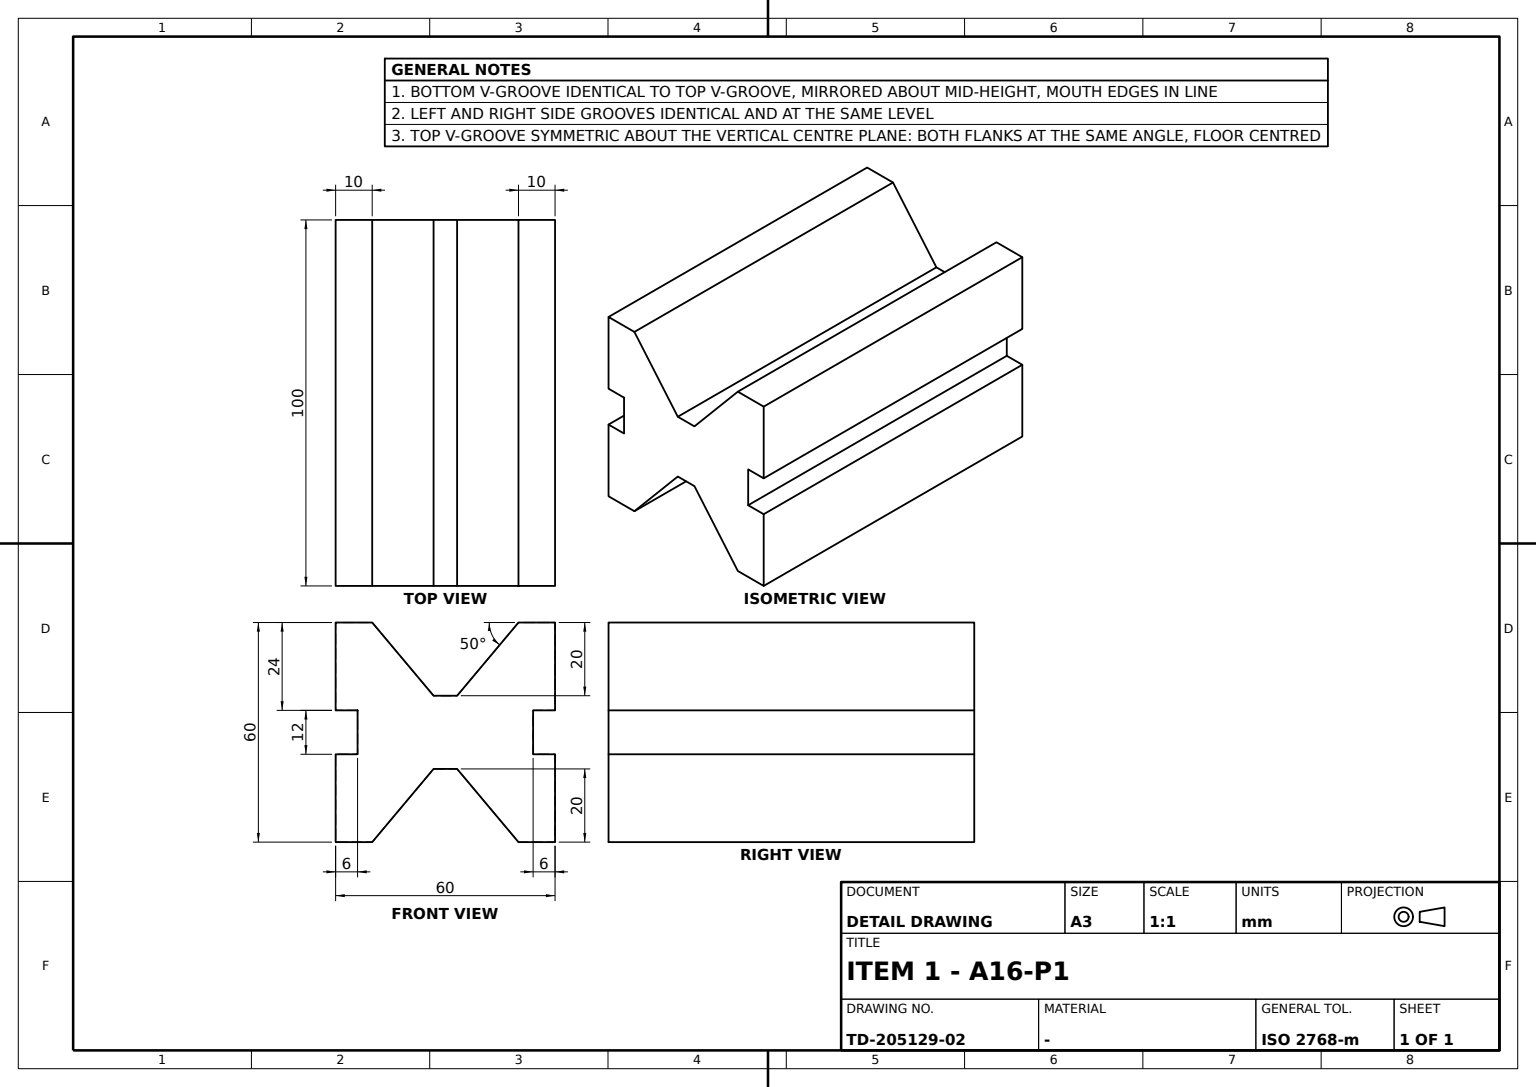
ISO-10303-21;
HEADER;
FILE_DESCRIPTION((''),'2;1');
FILE_NAME('','',(''),(''),'','','');
FILE_SCHEMA(('AUTOMOTIVE_DESIGN'));
ENDSEC;
DATA;
#1=APPLICATION_CONTEXT('');
#2=PRODUCT_CONTEXT('',#1,'mechanical');
#3=PRODUCT('','','',(#2));
#4=PRODUCT_DEFINITION_FORMATION('','',#3);
#5=PRODUCT_DEFINITION_CONTEXT('',#1,'design');
#6=PRODUCT_DEFINITION('','',#4,#5);
#7=PRODUCT_DEFINITION_SHAPE('','',#6);
#8=(LENGTH_UNIT()NAMED_UNIT(*)SI_UNIT(.MILLI.,.METRE.));
#9=(NAMED_UNIT(*)PLANE_ANGLE_UNIT()SI_UNIT($,.RADIAN.));
#10=(NAMED_UNIT(*)SI_UNIT($,.STERADIAN.)SOLID_ANGLE_UNIT());
#11=UNCERTAINTY_MEASURE_WITH_UNIT(LENGTH_MEASURE(0.005),#8,'distance_accuracy_value','');
#12=(GEOMETRIC_REPRESENTATION_CONTEXT(3)GLOBAL_UNCERTAINTY_ASSIGNED_CONTEXT((#11))GLOBAL_UNIT_ASSIGNED_CONTEXT((#8,#9,#10))REPRESENTATION_CONTEXT('',''));
#13=CARTESIAN_POINT('',(100.,30.,-6.));
#14=VERTEX_POINT('',#13);
#15=CARTESIAN_POINT('',(100.,24.,-6.));
#16=VERTEX_POINT('',#15);
#17=CARTESIAN_POINT('',(100.,0.,-6.));
#18=DIRECTION('',(0.,-1.,0.));
#19=VECTOR('',#18,1000.);
#20=LINE('',#17,#19);
#21=EDGE_CURVE('',#14,#16,#20,.T.);
#22=ORIENTED_EDGE('',*,*,#21,.F.);
#23=CARTESIAN_POINT('',(0.,30.,-6.));
#24=VERTEX_POINT('',#23);
#25=DIRECTION('',(1.,0.,0.));
#26=VECTOR('',#25,1000.);
#27=LINE('',#23,#26);
#28=EDGE_CURVE('',#24,#14,#27,.T.);
#29=ORIENTED_EDGE('',*,*,#28,.F.);
#30=CARTESIAN_POINT('',(0.,24.,-6.));
#31=VERTEX_POINT('',#30);
#32=CARTESIAN_POINT('',(0.,0.,-6.));
#33=LINE('',#32,#19);
#34=EDGE_CURVE('',#24,#31,#33,.T.);
#35=ORIENTED_EDGE('',*,*,#34,.T.);
#36=LINE('',#30,#26);
#37=EDGE_CURVE('',#31,#16,#36,.T.);
#38=ORIENTED_EDGE('',*,*,#37,.T.);
#39=EDGE_LOOP('',(#22,#29,#35,#38));
#40=FACE_BOUND('',#39,.T.);
#41=CARTESIAN_POINT('',(0.,-24.,-6.));
#42=DIRECTION('',(0.,0.,1.));
#43=AXIS2_PLACEMENT_3D('',#41,#42,#18);
#44=PLANE('',#43);
#45=ADVANCED_FACE('',(#40),#44,.T.);
#46=CARTESIAN_POINT('',(100.,-30.,-6.));
#47=VERTEX_POINT('',#46);
#48=CARTESIAN_POINT('',(100.,-30.,-30.));
#49=VERTEX_POINT('',#48);
#50=CARTESIAN_POINT('',(100.,-30.,0.));
#51=DIRECTION('',(0.,0.,-1.));
#52=VECTOR('',#51,1000.);
#53=LINE('',#50,#52);
#54=EDGE_CURVE('',#47,#49,#53,.T.);
#55=ORIENTED_EDGE('',*,*,#54,.F.);
#56=CARTESIAN_POINT('',(0.,-30.,-6.));
#57=VERTEX_POINT('',#56);
#58=LINE('',#56,#26);
#59=EDGE_CURVE('',#57,#47,#58,.T.);
#60=ORIENTED_EDGE('',*,*,#59,.F.);
#61=CARTESIAN_POINT('',(0.,-30.,-30.));
#62=VERTEX_POINT('',#61);
#63=CARTESIAN_POINT('',(0.,-30.,0.));
#64=LINE('',#63,#52);
#65=EDGE_CURVE('',#57,#62,#64,.T.);
#66=ORIENTED_EDGE('',*,*,#65,.T.);
#67=LINE('',#61,#26);
#68=EDGE_CURVE('',#62,#49,#67,.T.);
#69=ORIENTED_EDGE('',*,*,#68,.T.);
#70=EDGE_LOOP('',(#55,#60,#66,#69));
#71=FACE_BOUND('',#70,.T.);
#72=AXIS2_PLACEMENT_3D('',#56,#18,#51);
#73=PLANE('',#72);
#74=ADVANCED_FACE('',(#71),#73,.T.);
#75=CARTESIAN_POINT('',(0.,30.,30.));
#76=VERTEX_POINT('',#75);
#77=CARTESIAN_POINT('',(0.,30.,6.));
#78=VERTEX_POINT('',#77);
#79=CARTESIAN_POINT('',(0.,30.,-30.));
#80=LINE('',#79,#52);
#81=EDGE_CURVE('',#76,#78,#80,.T.);
#82=ORIENTED_EDGE('',*,*,#81,.F.);
#83=CARTESIAN_POINT('',(100.,30.,30.));
#84=VERTEX_POINT('',#83);
#85=LINE('',#75,#26);
#86=EDGE_CURVE('',#76,#84,#85,.T.);
#87=ORIENTED_EDGE('',*,*,#86,.T.);
#88=CARTESIAN_POINT('',(100.,30.,6.));
#89=VERTEX_POINT('',#88);
#90=CARTESIAN_POINT('',(100.,30.,-30.));
#91=LINE('',#90,#52);
#92=EDGE_CURVE('',#84,#89,#91,.T.);
#93=ORIENTED_EDGE('',*,*,#92,.T.);
#94=LINE('',#77,#26);
#95=EDGE_CURVE('',#78,#89,#94,.T.);
#96=ORIENTED_EDGE('',*,*,#95,.F.);
#97=EDGE_LOOP('',(#82,#87,#93,#96));
#98=FACE_BOUND('',#97,.T.);
#99=DIRECTION('',(0.,1.,0.));
#100=AXIS2_PLACEMENT_3D('',#79,#99,#42);
#101=PLANE('',#100);
#102=ADVANCED_FACE('',(#98),#101,.T.);
#103=VERTEX_POINT('',#41);
#104=CARTESIAN_POINT('',(100.,-24.,-6.));
#105=VERTEX_POINT('',#104);
#106=LINE('',#41,#26);
#107=EDGE_CURVE('',#103,#105,#106,.T.);
#108=ORIENTED_EDGE('',*,*,#107,.F.);
#109=EDGE_CURVE('',#103,#57,#33,.T.);
#110=ORIENTED_EDGE('',*,*,#109,.T.);
#111=ORIENTED_EDGE('',*,*,#59,.T.);
#112=EDGE_CURVE('',#105,#47,#20,.T.);
#113=ORIENTED_EDGE('',*,*,#112,.F.);
#114=EDGE_LOOP('',(#108,#110,#111,#113));
#115=FACE_BOUND('',#114,.T.);
#116=ADVANCED_FACE('',(#115),#44,.T.);
#117=CARTESIAN_POINT('',(0.,3.218007,10.));
#118=VERTEX_POINT('',#117);
#119=CARTESIAN_POINT('',(100.,3.218007,10.));
#120=VERTEX_POINT('',#119);
#121=LINE('',#117,#26);
#122=EDGE_CURVE('',#118,#120,#121,.T.);
#123=ORIENTED_EDGE('',*,*,#122,.F.);
#124=CARTESIAN_POINT('',(0.,-3.218007,10.));
#125=VERTEX_POINT('',#124);
#126=CARTESIAN_POINT('',(0.,0.,10.));
#127=VECTOR('',#99,1000.);
#128=LINE('',#126,#127);
#129=EDGE_CURVE('',#125,#118,#128,.T.);
#130=ORIENTED_EDGE('',*,*,#129,.F.);
#131=CARTESIAN_POINT('',(100.,-3.218007,10.));
#132=VERTEX_POINT('',#131);
#133=LINE('',#124,#26);
#134=EDGE_CURVE('',#125,#132,#133,.T.);
#135=ORIENTED_EDGE('',*,*,#134,.T.);
#136=CARTESIAN_POINT('',(100.,0.,10.));
#137=LINE('',#136,#127);
#138=EDGE_CURVE('',#132,#120,#137,.T.);
#139=ORIENTED_EDGE('',*,*,#138,.T.);
#140=EDGE_LOOP('',(#123,#130,#135,#139));
#141=FACE_BOUND('',#140,.T.);
#142=AXIS2_PLACEMENT_3D('',#124,#51,#99);
#143=PLANE('',#142);
#144=ADVANCED_FACE('',(#141),#143,.F.);
#145=ORIENTED_EDGE('',*,*,#122,.T.);
#146=CARTESIAN_POINT('',(100.,20.,30.));
#147=VERTEX_POINT('',#146);
#148=CARTESIAN_POINT('',(100.,-3.035635,2.5472));
#149=DIRECTION('',(0.,0.64278761,0.766044443));
#150=VECTOR('',#149,1000.);
#151=LINE('',#148,#150);
#152=EDGE_CURVE('',#120,#147,#151,.T.);
#153=ORIENTED_EDGE('',*,*,#152,.T.);
#154=CARTESIAN_POINT('',(0.,20.,30.));
#155=VERTEX_POINT('',#154);
#156=LINE('',#154,#26);
#157=EDGE_CURVE('',#155,#147,#156,.T.);
#158=ORIENTED_EDGE('',*,*,#157,.F.);
#159=CARTESIAN_POINT('',(0.,-3.035635,2.5472));
#160=LINE('',#159,#150);
#161=EDGE_CURVE('',#118,#155,#160,.T.);
#162=ORIENTED_EDGE('',*,*,#161,.F.);
#163=EDGE_LOOP('',(#145,#153,#158,#162));
#164=FACE_BOUND('',#163,.T.);
#165=DIRECTION('',(0.,0.766044443,-0.64278761));
#166=AXIS2_PLACEMENT_3D('',#117,#165,#149);
#167=PLANE('',#166);
#168=ADVANCED_FACE('',(#164),#167,.F.);
#169=CARTESIAN_POINT('',(0.,-30.,30.));
#170=VERTEX_POINT('',#169);
#171=CARTESIAN_POINT('',(100.,-30.,30.));
#172=VERTEX_POINT('',#171);
#173=LINE('',#169,#26);
#174=EDGE_CURVE('',#170,#172,#173,.T.);
#175=ORIENTED_EDGE('',*,*,#174,.T.);
#176=CARTESIAN_POINT('',(100.,-20.,30.));
#177=VERTEX_POINT('',#176);
#178=CARTESIAN_POINT('',(100.,0.,30.));
#179=LINE('',#178,#127);
#180=EDGE_CURVE('',#172,#177,#179,.T.);
#181=ORIENTED_EDGE('',*,*,#180,.T.);
#182=CARTESIAN_POINT('',(0.,-20.,30.));
#183=VERTEX_POINT('',#182);
#184=LINE('',#182,#26);
#185=EDGE_CURVE('',#183,#177,#184,.T.);
#186=ORIENTED_EDGE('',*,*,#185,.F.);
#187=CARTESIAN_POINT('',(0.,0.,30.));
#188=LINE('',#187,#127);
#189=EDGE_CURVE('',#170,#183,#188,.T.);
#190=ORIENTED_EDGE('',*,*,#189,.F.);
#191=EDGE_LOOP('',(#175,#181,#186,#190));
#192=FACE_BOUND('',#191,.T.);
#193=AXIS2_PLACEMENT_3D('',#154,#51,#99);
#194=PLANE('',#193);
#195=ADVANCED_FACE('',(#192),#194,.F.);
#196=CARTESIAN_POINT('',(100.,-24.,6.));
#197=VERTEX_POINT('',#196);
#198=CARTESIAN_POINT('',(100.,-30.,6.));
#199=VERTEX_POINT('',#198);
#200=CARTESIAN_POINT('',(100.,0.,6.));
#201=LINE('',#200,#19);
#202=EDGE_CURVE('',#197,#199,#201,.T.);
#203=ORIENTED_EDGE('',*,*,#202,.T.);
#204=CARTESIAN_POINT('',(0.,-30.,6.));
#205=VERTEX_POINT('',#204);
#206=LINE('',#204,#26);
#207=EDGE_CURVE('',#205,#199,#206,.T.);
#208=ORIENTED_EDGE('',*,*,#207,.F.);
#209=CARTESIAN_POINT('',(0.,-24.,6.));
#210=VERTEX_POINT('',#209);
#211=CARTESIAN_POINT('',(0.,0.,6.));
#212=LINE('',#211,#19);
#213=EDGE_CURVE('',#210,#205,#212,.T.);
#214=ORIENTED_EDGE('',*,*,#213,.F.);
#215=LINE('',#209,#26);
#216=EDGE_CURVE('',#210,#197,#215,.T.);
#217=ORIENTED_EDGE('',*,*,#216,.T.);
#218=EDGE_LOOP('',(#203,#208,#214,#217));
#219=FACE_BOUND('',#218,.T.);
#220=AXIS2_PLACEMENT_3D('',#77,#42,#18);
#221=PLANE('',#220);
#222=ADVANCED_FACE('',(#219),#221,.F.);
#223=ORIENTED_EDGE('',*,*,#68,.F.);
#224=CARTESIAN_POINT('',(0.,-20.,-30.));
#225=VERTEX_POINT('',#224);
#226=CARTESIAN_POINT('',(0.,0.,-30.));
#227=LINE('',#226,#127);
#228=EDGE_CURVE('',#62,#225,#227,.T.);
#229=ORIENTED_EDGE('',*,*,#228,.T.);
#230=CARTESIAN_POINT('',(100.,-20.,-30.));
#231=VERTEX_POINT('',#230);
#232=LINE('',#224,#26);
#233=EDGE_CURVE('',#225,#231,#232,.T.);
#234=ORIENTED_EDGE('',*,*,#233,.T.);
#235=CARTESIAN_POINT('',(100.,0.,-30.));
#236=LINE('',#235,#127);
#237=EDGE_CURVE('',#49,#231,#236,.T.);
#238=ORIENTED_EDGE('',*,*,#237,.F.);
#239=EDGE_LOOP('',(#223,#229,#234,#238));
#240=FACE_BOUND('',#239,.T.);
#241=AXIS2_PLACEMENT_3D('',#61,#51,#99);
#242=PLANE('',#241);
#243=ADVANCED_FACE('',(#240),#242,.T.);
#244=CARTESIAN_POINT('',(0.,20.,-30.));
#245=VERTEX_POINT('',#244);
#246=CARTESIAN_POINT('',(100.,20.,-30.));
#247=VERTEX_POINT('',#246);
#248=LINE('',#244,#26);
#249=EDGE_CURVE('',#245,#247,#248,.T.);
#250=ORIENTED_EDGE('',*,*,#249,.F.);
#251=VERTEX_POINT('',#79);
#252=EDGE_CURVE('',#245,#251,#227,.T.);
#253=ORIENTED_EDGE('',*,*,#252,.T.);
#254=VERTEX_POINT('',#90);
#255=LINE('',#79,#26);
#256=EDGE_CURVE('',#251,#254,#255,.T.);
#257=ORIENTED_EDGE('',*,*,#256,.T.);
#258=EDGE_CURVE('',#247,#254,#236,.T.);
#259=ORIENTED_EDGE('',*,*,#258,.F.);
#260=EDGE_LOOP('',(#250,#253,#257,#259));
#261=FACE_BOUND('',#260,.T.);
#262=ADVANCED_FACE('',(#261),#242,.T.);
#263=VECTOR('',#42,1000.);
#264=LINE('',#56,#263);
#265=EDGE_CURVE('',#205,#170,#264,.T.);
#266=ORIENTED_EDGE('',*,*,#265,.F.);
#267=ORIENTED_EDGE('',*,*,#207,.T.);
#268=LINE('',#46,#263);
#269=EDGE_CURVE('',#199,#172,#268,.T.);
#270=ORIENTED_EDGE('',*,*,#269,.T.);
#271=ORIENTED_EDGE('',*,*,#174,.F.);
#272=EDGE_LOOP('',(#266,#267,#270,#271));
#273=FACE_BOUND('',#272,.T.);
#274=ADVANCED_FACE('',(#273),#73,.T.);
#275=ORIENTED_EDGE('',*,*,#107,.T.);
#276=CARTESIAN_POINT('',(100.,-24.,0.));
#277=LINE('',#276,#52);
#278=EDGE_CURVE('',#197,#105,#277,.T.);
#279=ORIENTED_EDGE('',*,*,#278,.F.);
#280=ORIENTED_EDGE('',*,*,#216,.F.);
#281=CARTESIAN_POINT('',(0.,-24.,0.));
#282=LINE('',#281,#52);
#283=EDGE_CURVE('',#210,#103,#282,.T.);
#284=ORIENTED_EDGE('',*,*,#283,.T.);
#285=EDGE_LOOP('',(#275,#279,#280,#284));
#286=FACE_BOUND('',#285,.T.);
#287=AXIS2_PLACEMENT_3D('',#209,#18,#51);
#288=PLANE('',#287);
#289=ADVANCED_FACE('',(#286),#288,.T.);
#290=CARTESIAN_POINT('',(100.,24.,6.));
#291=VERTEX_POINT('',#290);
#292=EDGE_CURVE('',#89,#291,#201,.T.);
#293=ORIENTED_EDGE('',*,*,#292,.T.);
#294=CARTESIAN_POINT('',(0.,24.,6.));
#295=VERTEX_POINT('',#294);
#296=LINE('',#294,#26);
#297=EDGE_CURVE('',#295,#291,#296,.T.);
#298=ORIENTED_EDGE('',*,*,#297,.F.);
#299=EDGE_CURVE('',#78,#295,#212,.T.);
#300=ORIENTED_EDGE('',*,*,#299,.F.);
#301=ORIENTED_EDGE('',*,*,#95,.T.);
#302=EDGE_LOOP('',(#293,#298,#300,#301));
#303=FACE_BOUND('',#302,.T.);
#304=ADVANCED_FACE('',(#303),#221,.F.);
#305=CARTESIAN_POINT('',(0.,-3.218007,-10.));
#306=VERTEX_POINT('',#305);
#307=CARTESIAN_POINT('',(100.,-3.218007,-10.));
#308=VERTEX_POINT('',#307);
#309=LINE('',#305,#26);
#310=EDGE_CURVE('',#306,#308,#309,.T.);
#311=ORIENTED_EDGE('',*,*,#310,.F.);
#312=CARTESIAN_POINT('',(0.,3.218007,-10.));
#313=VERTEX_POINT('',#312);
#314=CARTESIAN_POINT('',(0.,0.,-10.));
#315=LINE('',#314,#127);
#316=EDGE_CURVE('',#306,#313,#315,.T.);
#317=ORIENTED_EDGE('',*,*,#316,.T.);
#318=CARTESIAN_POINT('',(100.,3.218007,-10.));
#319=VERTEX_POINT('',#318);
#320=LINE('',#312,#26);
#321=EDGE_CURVE('',#313,#319,#320,.T.);
#322=ORIENTED_EDGE('',*,*,#321,.T.);
#323=CARTESIAN_POINT('',(100.,0.,-10.));
#324=LINE('',#323,#127);
#325=EDGE_CURVE('',#308,#319,#324,.T.);
#326=ORIENTED_EDGE('',*,*,#325,.F.);
#327=EDGE_LOOP('',(#311,#317,#322,#326));
#328=FACE_BOUND('',#327,.T.);
#329=AXIS2_PLACEMENT_3D('',#305,#51,#99);
#330=PLANE('',#329);
#331=ADVANCED_FACE('',(#328),#330,.T.);
#332=EDGE_CURVE('',#155,#76,#188,.T.);
#333=ORIENTED_EDGE('',*,*,#332,.F.);
#334=ORIENTED_EDGE('',*,*,#157,.T.);
#335=EDGE_CURVE('',#147,#84,#179,.T.);
#336=ORIENTED_EDGE('',*,*,#335,.T.);
#337=ORIENTED_EDGE('',*,*,#86,.F.);
#338=EDGE_LOOP('',(#333,#334,#336,#337));
#339=FACE_BOUND('',#338,.T.);
#340=ADVANCED_FACE('',(#339),#194,.F.);
#341=CARTESIAN_POINT('',(100.,3.035635,2.5472));
#342=DIRECTION('',(0.,0.64278761,-0.766044443));
#343=VECTOR('',#342,1000.);
#344=LINE('',#341,#343);
#345=EDGE_CURVE('',#177,#132,#344,.T.);
#346=ORIENTED_EDGE('',*,*,#345,.T.);
#347=ORIENTED_EDGE('',*,*,#134,.F.);
#348=CARTESIAN_POINT('',(0.,3.035635,2.5472));
#349=LINE('',#348,#343);
#350=EDGE_CURVE('',#183,#125,#349,.T.);
#351=ORIENTED_EDGE('',*,*,#350,.F.);
#352=ORIENTED_EDGE('',*,*,#185,.T.);
#353=EDGE_LOOP('',(#346,#347,#351,#352));
#354=FACE_BOUND('',#353,.T.);
#355=DIRECTION('',(0.,-0.766044443,-0.64278761));
#356=AXIS2_PLACEMENT_3D('',#182,#355,#342);
#357=PLANE('',#356);
#358=ADVANCED_FACE('',(#354),#357,.F.);
#359=ORIENTED_EDGE('',*,*,#28,.T.);
#360=CARTESIAN_POINT('',(100.,30.,0.));
#361=LINE('',#360,#263);
#362=EDGE_CURVE('',#254,#14,#361,.T.);
#363=ORIENTED_EDGE('',*,*,#362,.F.);
#364=ORIENTED_EDGE('',*,*,#256,.F.);
#365=CARTESIAN_POINT('',(0.,30.,0.));
#366=LINE('',#365,#263);
#367=EDGE_CURVE('',#251,#24,#366,.T.);
#368=ORIENTED_EDGE('',*,*,#367,.T.);
#369=EDGE_LOOP('',(#359,#363,#364,#368));
#370=FACE_BOUND('',#369,.T.);
#371=ADVANCED_FACE('',(#370),#101,.T.);
#372=CARTESIAN_POINT('',(100.,-3.035635,-2.5472));
#373=LINE('',#372,#343);
#374=EDGE_CURVE('',#319,#247,#373,.T.);
#375=ORIENTED_EDGE('',*,*,#374,.T.);
#376=ORIENTED_EDGE('',*,*,#258,.T.);
#377=ORIENTED_EDGE('',*,*,#362,.T.);
#378=ORIENTED_EDGE('',*,*,#21,.T.);
#379=CARTESIAN_POINT('',(100.,24.,0.));
#380=LINE('',#379,#263);
#381=EDGE_CURVE('',#16,#291,#380,.T.);
#382=ORIENTED_EDGE('',*,*,#381,.T.);
#383=ORIENTED_EDGE('',*,*,#292,.F.);
#384=ORIENTED_EDGE('',*,*,#92,.F.);
#385=ORIENTED_EDGE('',*,*,#335,.F.);
#386=ORIENTED_EDGE('',*,*,#152,.F.);
#387=ORIENTED_EDGE('',*,*,#138,.F.);
#388=ORIENTED_EDGE('',*,*,#345,.F.);
#389=ORIENTED_EDGE('',*,*,#180,.F.);
#390=ORIENTED_EDGE('',*,*,#269,.F.);
#391=ORIENTED_EDGE('',*,*,#202,.F.);
#392=ORIENTED_EDGE('',*,*,#278,.T.);
#393=ORIENTED_EDGE('',*,*,#112,.T.);
#394=ORIENTED_EDGE('',*,*,#54,.T.);
#395=ORIENTED_EDGE('',*,*,#237,.T.);
#396=CARTESIAN_POINT('',(100.,3.035635,-2.5472));
#397=LINE('',#396,#150);
#398=EDGE_CURVE('',#231,#308,#397,.T.);
#399=ORIENTED_EDGE('',*,*,#398,.T.);
#400=ORIENTED_EDGE('',*,*,#325,.T.);
#401=EDGE_LOOP('',(#375,#376,#377,#378,#382,#383,#384,#385,#386,#387,#388,#389,#390,#391,#392,#393,#394,#395,#399,#400));
#402=FACE_BOUND('',#401,.T.);
#403=CARTESIAN_POINT('',(100.,0.,0.));
#404=AXIS2_PLACEMENT_3D('',#403,#25,#99);
#405=PLANE('',#404);
#406=ADVANCED_FACE('',(#402),#405,.T.);
#407=CARTESIAN_POINT('',(0.,3.035635,-2.5472));
#408=LINE('',#407,#150);
#409=EDGE_CURVE('',#225,#306,#408,.T.);
#410=ORIENTED_EDGE('',*,*,#409,.T.);
#411=ORIENTED_EDGE('',*,*,#310,.T.);
#412=ORIENTED_EDGE('',*,*,#398,.F.);
#413=ORIENTED_EDGE('',*,*,#233,.F.);
#414=EDGE_LOOP('',(#410,#411,#412,#413));
#415=FACE_BOUND('',#414,.T.);
#416=AXIS2_PLACEMENT_3D('',#224,#165,#149);
#417=PLANE('',#416);
#418=ADVANCED_FACE('',(#415),#417,.T.);
#419=ORIENTED_EDGE('',*,*,#249,.T.);
#420=ORIENTED_EDGE('',*,*,#374,.F.);
#421=ORIENTED_EDGE('',*,*,#321,.F.);
#422=CARTESIAN_POINT('',(0.,-3.035635,-2.5472));
#423=LINE('',#422,#343);
#424=EDGE_CURVE('',#313,#245,#423,.T.);
#425=ORIENTED_EDGE('',*,*,#424,.T.);
#426=EDGE_LOOP('',(#419,#420,#421,#425));
#427=FACE_BOUND('',#426,.T.);
#428=AXIS2_PLACEMENT_3D('',#312,#355,#342);
#429=PLANE('',#428);
#430=ADVANCED_FACE('',(#427),#429,.T.);
#431=ORIENTED_EDGE('',*,*,#332,.T.);
#432=ORIENTED_EDGE('',*,*,#81,.T.);
#433=ORIENTED_EDGE('',*,*,#299,.T.);
#434=CARTESIAN_POINT('',(0.,24.,0.));
#435=LINE('',#434,#263);
#436=EDGE_CURVE('',#31,#295,#435,.T.);
#437=ORIENTED_EDGE('',*,*,#436,.F.);
#438=ORIENTED_EDGE('',*,*,#34,.F.);
#439=ORIENTED_EDGE('',*,*,#367,.F.);
#440=ORIENTED_EDGE('',*,*,#252,.F.);
#441=ORIENTED_EDGE('',*,*,#424,.F.);
#442=ORIENTED_EDGE('',*,*,#316,.F.);
#443=ORIENTED_EDGE('',*,*,#409,.F.);
#444=ORIENTED_EDGE('',*,*,#228,.F.);
#445=ORIENTED_EDGE('',*,*,#65,.F.);
#446=ORIENTED_EDGE('',*,*,#109,.F.);
#447=ORIENTED_EDGE('',*,*,#283,.F.);
#448=ORIENTED_EDGE('',*,*,#213,.T.);
#449=ORIENTED_EDGE('',*,*,#265,.T.);
#450=ORIENTED_EDGE('',*,*,#189,.T.);
#451=ORIENTED_EDGE('',*,*,#350,.T.);
#452=ORIENTED_EDGE('',*,*,#129,.T.);
#453=ORIENTED_EDGE('',*,*,#161,.T.);
#454=EDGE_LOOP('',(#431,#432,#433,#437,#438,#439,#440,#441,#442,#443,#444,#445,#446,#447,#448,#449,#450,#451,#452,#453));
#455=FACE_BOUND('',#454,.T.);
#456=CARTESIAN_POINT('',(0.,0.,0.));
#457=AXIS2_PLACEMENT_3D('',#456,#25,#99);
#458=PLANE('',#457);
#459=ADVANCED_FACE('',(#455),#458,.F.);
#460=ORIENTED_EDGE('',*,*,#297,.T.);
#461=ORIENTED_EDGE('',*,*,#381,.F.);
#462=ORIENTED_EDGE('',*,*,#37,.F.);
#463=ORIENTED_EDGE('',*,*,#436,.T.);
#464=EDGE_LOOP('',(#460,#461,#462,#463));
#465=FACE_BOUND('',#464,.T.);
#466=AXIS2_PLACEMENT_3D('',#30,#99,#42);
#467=PLANE('',#466);
#468=ADVANCED_FACE('',(#465),#467,.T.);
#469=CLOSED_SHELL('',(#45,#74,#102,#116,#144,#168,#195,#222,#243,#262,#274,#289,#304,#331,#340,#358,#371,#406,#418,#430,#459,#468));
#470=MANIFOLD_SOLID_BREP('',#469);
#471=ADVANCED_BREP_SHAPE_REPRESENTATION('',(#470),#12);
#472=SHAPE_DEFINITION_REPRESENTATION(#7,#471);
ENDSEC;
END-ISO-10303-21;
